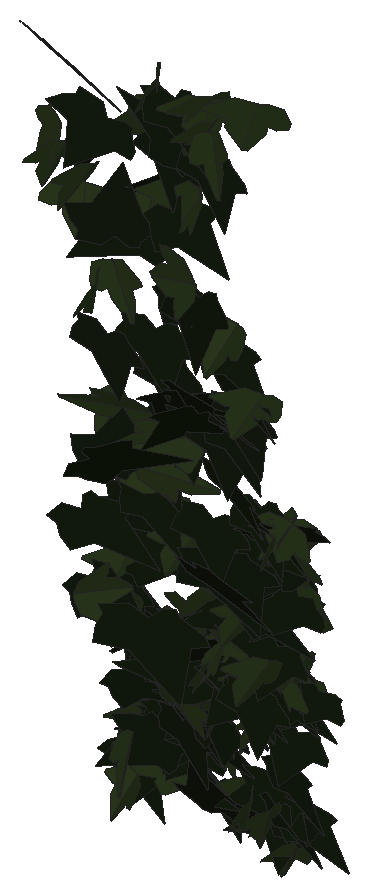
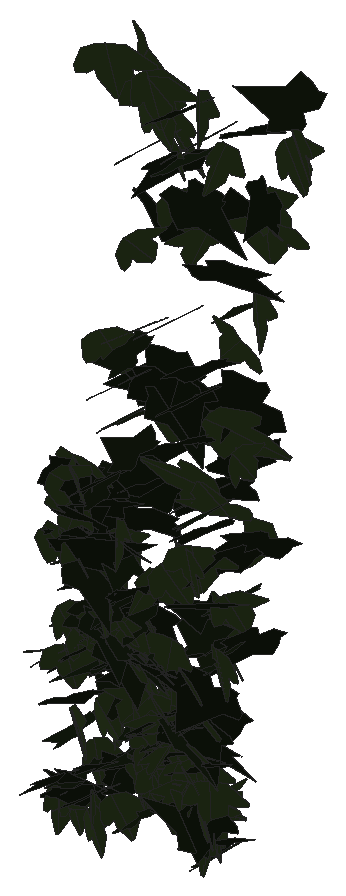
# SketchUp Ruby script. Lengths in millimetres.
U = 1.mm
M = Sketchup.active_model
def pt(a) = Geom::Point3d.new(a.map { |v| v * U })
def face(e, loops, mat)
  f = e.add_face(loops[0].map { |a| pt(a) })
  loops[1..].each { |l| e.add_face(l.map { |a| pt(a) }).erase! }
  f.material = f.back_material = mat if mat
  f
end
# faces: each face lists its corners as indices into pts; further lists are holes
def faces(e, pts, list, mat = nil) = list.each { |f| face(e, (f[0].is_a?(Array) ? f : [f]).map { |l| l.map { |i| pts[i] } }, mat) }
# xy, xz, yz: faces in a plane at the given z, y or x. An outline is a flat list of corners, or four numbers for a rectangle; further outlines are holes
def ring(l) = l.size == 4 ? [[l[0], l[1]], [l[2], l[1]], [l[2], l[3]], [l[0], l[3]]] : l.each_slice(2).to_a
def flat(e, list, mat, &to3) = list.each { |f| face(e, (f[0].is_a?(Array) ? f : [f]).map { |l| ring(l).map { |u, v| to3.(u, v) } }, mat) }
def xy(e, z, list, mat = nil) = flat(e, list, mat) { |x, y| [x, y, z] }
def xz(e, y, list, mat = nil) = flat(e, list, mat) { |x, z| [x, y, z] }
def yz(e, x, list, mat = nil) = flat(e, list, mat) { |y, z| [x, y, z] }
def lines(e, pts, list) = list.each { |a, b| e.add_line(pt(pts[a]), pt(pts[b])) }
# prism: a flat outline (further loops are holes) pulled along v
def prism(e, loops, v, mat = nil)
  f = face(e, loops, mat); d = Geom::Vector3d.new(v.map { |x| x * U })
  f.pushpull(f.normal.samedirection?(d) ? d.length : -d.length)
end
def box(e, o, s, mat = nil) = prism(e, [[o, [o[0] + s[0], o[1], o[2]], [o[0] + s[0], o[1] + s[1], o[2]], [o[0], o[1] + s[1], o[2]]]], [0, 0, s[2]], mat)
def at(x, y, z, deg = 0) = Geom::Transformation.translation(pt([x, y, z])) * Geom::Transformation.rotation(ORIGIN, Z_AXIS, deg.degrees)
def axes(o, x, y, z) = Geom::Transformation.new([*x, 0, *y, 0, *z, 0, *pt(o).to_a, 1])
def part(name) = M.definitions.add(name)
# library, detail: a bought-in or finely detailed component or shape, given as its bounding box
def library(name, o, s) = part(name).tap { |d| box(d.entities, o, s) }
def detail(e, o, s) = box(e.add_group.entities, o, s)
def put(e, d, t, mat = nil) = e.add_instance(d, t).tap { |i| i.material = mat if mat }
def group(e, t, mat = nil) = e.add_group.tap { |g| g.transformation = t; g.material = mat if mat }.entities
root = M.entities
M.materials.add("efeu1").color = [18, 25, 13]
M.materials.add("efeu2").color = [43, 57, 29]
c1 = part("ivyleaf_10")
p = [[0,12.8,-0.8],[-1.5,51.3,-10.9],[-4.9,51,-11.6],[-13.6,26.5,-7.3],[-13.2,15.9,-4.6],[-21.1,19.3,-7.2],
  [-29.5,16.3,-8.3],[-29.2,8.3,-6.2],[-19.7,-9.8,0.5],[-7.6,-13,4],[1,-12.2,5.8],[-0.4,51.1,-11.1],
  [-1.5,51.1,-10.9],[1,-12.4,5.9],[16.9,-12.4,3.5],[35.1,9.1,-5.1],[35,12.9,-6.1],[20.5,16.4,-4.9],
  [15.8,15,-3.8],[15.3,27.6,-7.1],[12.8,31.3,-7.8]]
faces(c1.entities,p,[[0,1,2,3,4,5,6,7,8,9,10],[11,12,0,13,14,15,16,17,18,19,20]],"efeu2")
c2 = part("ivyleaf_9")
p = [[39.1,54.8,31.7],[34.5,51.8,30.2],[-5.3,25.2,17.3],[-17.9,28.3,20.9],[-21.6,21.7,17],[-20.2,4.3,5.3],
  [-22.9,-0.3,2.5],[-17.1,-4,-0.6],[-2,-2.1,-1.2],[-0.7,-15.4,-10.1],[16.6,-22.3,-16.7],[21.1,-15.1,-12.5],
  [32.7,-10.7,-11],[46.1,-1.8,-6.6],[30.8,11.2,3.8]]
faces(c2.entities,p,[[0,1,2,3,4,5,6,7,8,9,10,11,12,13,14]],"efeu1")
put(root,c1,axes([1434.4,970.3,1660.3],[-1.04964,0.5725,0.28622],[-0.43851,0.17492,-0.79383],[-1.1365,-0.59623,0.04194]))
put(root,c2,axes([1417.1,894.4,1905.8],[0.23864,-0.56618,-0.78224],[-0.27175,0.76926,-0.57968],[1.8176,0.18935,0.01604]))
put(root,c2,axes([1415.3,969.2,1644.3],[0.27967,-0.82614,-0.05758],[-0.01819,0.05678,-0.83911],[1.57602,0.14726,0.00053]))
put(root,c1,axes([1435.7,960,1718.2],[-1.01449,-0.6751,-0.06263],[0.06682,0.05208,-0.86016],[1.28864,-0.53418,-0.0047]))
put(root,c1,axes([1431.5,964.2,1672.8],[0.35686,-0.82142,0.0966],[0.12958,-0.08338,-0.84121],[1.56876,0.19375,0.04751]))
put(root,c2,axes([1429.2,970.8,1655.9],[-0.76095,-0.73239,0.12628],[0.0387,-0.15413,-0.82948],[1.41392,-0.38994,0.09067]))
put(root,c2,axes([1396.9,838,2598.5],[0.91673,-0.76677,0.5409],[0.7383,-0.3909,-0.89958],[1.62613,0.60974,0.1035]))
put(root,c1,axes([1433.1,943.4,1890.3],[1.07356,-0.65991,-0.22821],[0.00287,0.29452,-0.84794],[1.32891,0.53247,0.18619]))
put(root,c2,axes([1442.1,845.9,2471],[-0.26448,0.20363,-0.96166],[-1.08746,0.77356,0.24637],[1.5223,0.58798,0.00891]))
put(root,c1,axes([1441.2,790,2530.7],[0.91565,-0.84518,-0.38706],[-0.21709,0.37886,-0.96906],[1.75584,0.4876,0.08203]))
put(root,c1,axes([1438,968.2,1685.2],[0.3553,-0.82918,0.02072],[0.01414,-0.01956,-0.84994],[1.57853,0.18681,0.00295]))
put(root,c1,axes([1444.9,957.2,1685.3],[-0.56888,-0.76943,0.24282],[-0.09597,-0.24063,-0.82455],[1.53256,-0.30068,0.0385]))
put(root,c1,axes([1445.2,840.3,2455],[-0.07469,-0.99115,0.30908],[-0.05688,-0.30809,-0.99178],[1.97513,-0.04635,-0.01687]))
put(root,c1,axes([1446.4,793.8,2506.2],[-0.23783,-1.02613,0.13782],[0.04918,-0.14187,-1.03284],[1.96986,-0.12035,0.04243]))
put(root,c1,axes([1439.1,900.2,2138.7],[-0.19002,-0.7118,0.60771],[0.39442,-0.6128,-0.68372],[1.73705,0.06128,0.22173]))
put(root,c2,axes([1447.4,964.6,1693.6],[0.96749,0.62386,-0.24385],[-0.49824,-0.09672,-0.79322],[-1.17341,0.55545,0.13575]))
put(root,c1,axes([1451.5,901.3,1940.8],[-0.72211,-0.75499,0.40283],[0.11994,-0.46411,-0.81048],[1.62421,-0.30139,0.23894]))
put(root,c1,axes([1441.6,842.8,2424],[1.7773,0.33849,0.00534],[0.00811,0.00391,-0.9933],[-0.64424,0.93386,0.00222]))
put(root,c2,axes([1436.8,899.8,2012.8],[0.5542,-0.31754,-0.82236],[-0.35804,0.82372,-0.38468],[1.63909,0.2873,0.19402]))
put(root,c2,axes([1443.1,948.5,1850.1],[1.40022,0.45952,-0.05842],[-0.09682,-0.02883,-0.86743],[-0.87627,0.73747,0.00249]))
put(root,c1,axes([1487.6,870.2,2154.6],[0.4405,0.36401,-0.91335],[-1.86951,0.12612,-0.19866],[0.08078,0.93374,0.3829]))
put(root,c1,axes([1458.6,839.2,2313.9],[0.18528,-0.93087,-0.39747],[0.05517,0.40171,-0.93369],[1.92559,0.07806,0.065]))
put(root,c1,axes([1460,954,1736.2],[-0.91075,-0.72045,-0.03433],[0.07,0.01677,-0.86464],[1.37094,-0.47947,0.02135]))
put(root,c2,axes([1433.3,857.4,2014.5],[0.29722,-0.55902,-0.7958],[0.35513,0.80824,-0.53115],[1.81652,-0.06654,0.23405]))
put(root,c2,axes([1441.5,973.3,1666.6],[0.20326,0.8293,-0.08372],[0.05259,0.08083,0.83598],[1.58548,-0.109,-0.01699]))
put(root,c1,axes([1436.5,902.7,2297.3],[1.35088,-0.33728,0.56936],[1.03127,-0.18308,-0.78396],[0.72299,0.89132,0.05442]))
put(root,c2,axes([1441.7,930.8,1886.7],[0.26193,-0.86894,0.15465],[0.05449,-0.15204,-0.87976],[1.67887,0.1405,0.00443]))
put(root,c2,axes([1446.7,949.7,1809.2],[0.32729,-0.86263,-0.07627],[-0.03067,0.07456,-0.87961],[1.64789,0.17272,-0.00122]))
put(root,c2,axes([1486.9,892,2377.5],[-1.65754,-0.3691,0.27433],[-0.49297,-0.09177,-0.94578],[0.72323,-0.90849,-0.01592]))
put(root,c2,axes([1478.5,939.4,1782.8],[0.29328,0.79954,-0.30007],[-0.29361,-0.27384,-0.80887],[-1.59859,0.19698,0.09351]))
put(root,c1,axes([1472.3,957.7,1698.3],[-0.92655,-0.69222,0.04256],[-0.03708,-0.03833,-0.84625],[1.3194,-0.48719,0.0061]))
put(root,c1,axes([1496,935,1675.2],[0.19709,0.03091,-0.87008],[-1.64931,-0.08056,-0.106],[-0.15927,0.87251,0.02104]))
put(root,c2,axes([1466.5,965.1,1737],[-0.73514,-0.74123,0.18677],[-0.17365,-0.16306,-0.83582],[1.4444,-0.39686,-0.00543]))
put(root,c2,axes([1488.2,960.4,1782.7],[-0.83597,0.74291,-0.00144],[0.00586,0.00015,-0.86304],[-1.4139,-0.43925,-0.00273]))
put(root,c1,axes([1472.1,963.3,1733],[-0.87648,-0.7133,-0.13305],[0.18693,0.09486,-0.84849],[1.36825,-0.46989,0.03069]))
put(root,c1,axes([1465.8,894.8,1666.3],[-0.2456,-0.44674,0.81263],[0.51462,-0.80293,-0.39847],[1.6882,0.17977,0.23969]))
put(root,c2,axes([1474.5,940.5,1948.6],[-1.1317,-0.64309,0.21061],[0.00802,-0.28389,-0.85492],[1.28787,-0.56334,0.1904]))
put(root,c2,axes([1457,912.2,1796.5],[0.15487,-0.18572,-0.95521],[-0.06411,0.95743,-0.18902],[1.85089,0.0487,0.07338]))
put(root,c1,axes([1480.8,935.1,2009.9],[-1.28263,-0.59584,0.15556],[0.02437,-0.24412,-0.87957],[1.17175,-0.64714,0.18857]))
put(root,c1,axes([1471.4,965.9,1714.4],[0.50447,0.78867,0.19855],[0.01441,0.20643,-0.83007],[-1.54777,0.25898,0.05699]))
put(root,c2,axes([1482.8,829.5,2538.4],[-1.0304,-0.75563,0.39473],[-0.24607,-0.38942,-0.92279],[1.60375,-0.54524,0.11202]))
put(root,c2,axes([1477,844.4,2095.4],[-0.86528,-0.37518,0.81195],[1.29354,0.44717,0.5872],[-1.10659,0.81608,0.05152]))
put(root,c2,axes([1462.6,929.5,2072],[0.40961,-0.88862,-0.13844],[-0.01827,0.14007,-0.91402],[1.71153,0.21417,0.02338]))
put(root,c1,axes([1481.6,949,1850.4],[0.9459,-0.73368,0.01446],[0.02477,-0.00865,-0.88615],[1.39639,0.49714,0.00592]))
put(root,c2,axes([1465.3,878.6,1929.5],[0.09638,-0.90044,0.13314],[0.08654,-0.13068,-0.90108],[1.7302,0.0567,0.03766]))
put(root,c1,axes([1467.9,894.7,2057.6],[1.66542,0.12632,-0.31002],[0.5173,0.23843,0.86434],[0.37194,-0.89722,0.18604]))
put(root,c1,axes([1481.6,876,2525.4],[-0.29444,-0.76586,-0.63412],[0.42807,0.59816,-0.7773],[1.84331,-0.26124,0.07922]))
put(root,c2,axes([1470.1,944.1,1854.7],[-0.03623,-0.8479,0.2664],[0.14076,-0.26705,-0.84468],[1.68563,0.00408,0.07626]))
put(root,c1,axes([1490.8,954.4,1688.4],[-1.35071,-0.4691,-0.00957],[0.01554,0.005,-0.85073],[0.89284,-0.70975,0.00033]))
put(root,c1,axes([1473.2,960.6,1731.9],[0.97081,-0.51401,0.45366],[0.64493,-0.30252,-0.72379],[1.13426,0.61195,0.02325]))
put(root,c2,axes([1498.2,954.2,1743.3],[-1.38987,-0.41323,0.17129],[-0.16559,-0.19045,-0.8304],[0.83508,-0.72552,0.12042]))
put(root,c2,axes([1510.6,894.3,1736.5],[-1.64683,0.01971,0.04934],[-0.09342,0.01165,-0.86545],[-0.03871,-0.86662,-0.01051]))
put(root,c2,axes([1472.1,946.1,1800.7],[0.41559,-0.83992,-0.13754],[0.05075,0.14867,-0.86559],[1.61902,0.21094,0.06244]))
put(root,c1,axes([1465.2,884.4,1899.4],[0.82946,-0.26126,0.83715],[1.45325,-0.34669,-0.50572],[0.82083,0.87782,0.04942]))
put(root,c1,axes([1498.4,930.9,2004.9],[1.07405,-0.68067,-0.24253],[-0.16028,0.24368,-0.87985],[1.36586,0.56385,0.08747]))
put(root,c1,axes([1491.8,956.9,1760.9],[1.62328,-0.14206,-0.02323],[-0.04513,-0.00095,-0.86466],[0.27022,0.85324,-0.00483]))
put(root,c2,axes([1479.1,919.9,2083.7],[0.2075,-0.92058,-0.06337],[0.01437,0.0647,-0.92689],[1.75614,0.10824,0.01507]))
put(root,c1,axes([1498.3,936.6,1785.3],[-1.52837,-0.32335,-0.1119],[0.19436,0.04596,-0.8657],[0.62153,-0.80951,-0.00446]))
put(root,c2,axes([1498.1,828.2,2401.8],[-1.21499,-0.40319,0.70228],[1.20254,0.3113,0.7531],[-0.96392,0.89657,0.05433]))
put(root,c1,axes([1494,788.4,1960.7],[0.06546,0.13379,1.09212],[-0.13984,1.09049,-0.13128],[-2.08938,-0.06879,0.043]))
put(root,c2,axes([1483.4,907.7,2035],[0.11537,-0.8883,-0.25008],[0.03162,0.25162,-0.88977],[1.75604,0.05383,0.03245]))
put(root,c2,axes([1501.5,956,1724.2],[-0.92501,-0.68308,0.11872],[-0.09382,-0.11057,-0.83801],[1.31619,-0.48795,0.0237]))
put(root,c1,axes([1507.5,966.8,1716.4],[-0.95439,-0.66753,0.15686],[-0.05818,-0.17238,-0.83128],[1.30375,-0.49635,0.07774]))
put(root,c2,axes([1480.7,899.8,1882.1],[0.40991,-0.81471,0.45489],[0.41271,-0.41037,-0.83764],[1.72725,0.2914,0.09219]))
put(root,c2,axes([1525.6,884.9,2458.9],[-0.53775,0.7891,-0.54165],[-0.00776,-0.56575,-0.82208],[-1.82156,-0.23055,0.16341]))
put(root,c2,axes([1507,962.7,1702.3],[-0.93225,-0.60352,0.33809],[-0.02156,-0.40721,-0.74332],[1.31639,-0.43407,0.22725]))
put(root,c1,axes([1513,943.9,1879.4],[-1.4834,0.38853,0.11578],[-0.23402,0.01252,-0.86982],[-0.73524,-0.78787,0.04327]))
put(root,c1,axes([1502.4,964.6,1752.3],[0.08807,0.85295,0.0692],[0.01301,0.06893,-0.8542],[-1.62862,0.04668,-0.00308]))
put(root,c1,axes([1515.7,938.5,1974.7],[-0.69758,-0.77477,0.4371],[-0.02028,-0.46889,-0.84006],[1.6929,-0.32487,0.17005]))
put(root,c1,axes([1501.3,890,2416.1],[0.6171,0.92853,0.11872],[0.02467,0.12118,-0.98313],[-1.7814,0.32333,0.02751]))
put(root,c2,axes([1498.7,901,2244.4],[-0.32905,-0.9389,-0.10082],[0.05503,0.09719,-0.95463],[1.79635,-0.17496,0.01078]))
put(root,c2,axes([1492.9,853.7,1870.9],[0.24376,0.95405,-0.29052],[-0.02416,0.29444,0.96133],[1.8979,-0.11879,0.04955]))
put(root,c2,axes([1508.7,947.7,1792.8],[-0.38927,-0.85126,0.02522],[-0.03907,-0.021,-0.87536],[1.62035,-0.20501,-0.01505]))
put(root,c2,axes([1502.7,960.2,1776.1],[-0.32992,-0.84195,-0.0494],[0.36895,0.0093,-0.83887],[1.56219,-0.18001,0.18769]))
put(root,c2,axes([1502.8,809.3,2280.3],[-0.14087,-0.94076,0.22442],[0.10811,-0.22892,-0.94088],[1.83753,-0.05865,0.07256]))
put(root,c1,axes([1520,869.5,2580.7],[0.15772,-0.88455,-0.49433],[0.12164,0.49955,-0.88318],[1.92468,0.04091,0.09633]))
put(root,c1,axes([1510.1,957,1785.8],[0.89566,0.7276,0.02766],[0.04432,0.01788,-0.86647],[-1.38505,0.47108,-0.00984]))
put(root,c2,axes([1507.7,911,2200.4],[-0.05042,-0.94817,0.06026],[-0.05488,-0.05946,-0.94815],[1.80736,-0.02826,-0.02711]))
put(root,c2,axes([1539.9,936.1,1853.5],[-1.31199,0.51075,-0.19193],[0.19098,-0.1853,-0.85353],[-1.02071,-0.69117,0.087]))
put(root,c1,axes([1551.2,870,2140.1],[0.9072,0.19364,-0.82272],[-1.51761,-0.21014,-0.51146],[-0.53333,0.92733,0.0559]))
put(root,c1,axes([1522.1,911.7,1783.9],[-1.40217,0.41996,-0.20628],[0.36595,-0.07902,-0.84764],[-0.8118,-0.76099,-0.02582]))
put(root,c2,axes([1516.8,957.9,1782.6],[-0.10107,-0.86174,-0.09082],[-0.01354,0.09142,-0.86328],[1.64908,-0.05206,-0.01265]))
put(root,c2,axes([1506.8,780.4,2139.5],[0.23389,0.59882,-0.92124],[0.20572,0.9159,0.60977],[2.08102,-0.15785,0.04326]))
put(root,c1,axes([1523.3,957.5,1813.6],[0.88738,-0.59261,0.43719],[0.47881,-0.35815,-0.75376],[1.31724,0.5294,-0.02054]))
put(root,c2,axes([1521.3,917.2,2139],[-0.31425,-0.92005,-0.12111],[0.03514,0.11973,-0.93474],[1.76579,-0.16612,-0.00295]))
put(root,c2,axes([1549.5,880.5,2504.4],[-0.44035,-0.96646,0.15669],[0.0664,0.15277,0.99377],[-1.86221,0.23398,-0.00162]))
put(root,c1,axes([1537.2,946.6,1760.8],[-0.73363,-0.74939,0.19121],[0.06349,-0.22955,-0.83242],[1.47056,-0.36394,0.13133]))
put(root,c1,axes([1538.3,949.8,1728.8],[-0.29447,-0.8501,0.0923],[0.01137,-0.09487,-0.86376],[1.62738,-0.15316,0.02274]))
put(root,c2,axes([1547.3,880.8,2170.9],[0.08015,0.93106,-0.20242],[-0.09256,-0.20026,-0.93122],[-1.81103,0.05144,0.03863]))
put(root,c1,axes([1541.7,887.6,2445.3],[-0.75847,-0.83351,0.36406],[-0.00462,-0.3965,-0.91043],[1.73105,-0.36627,0.15709]))
put(root,c2,axes([1517.1,945.1,1758.5],[0.3915,-0.83275,0.17944],[0.10617,-0.17104,-0.85769],[1.6178,0.21275,0.01286]))
put(root,c2,axes([1564.8,897.2,1830.9],[-1.08381,0.06456,0.67096],[-1.1579,-0.42736,-0.47525],[0.55227,-0.76931,0.32031]))
put(root,c1,axes([1502.7,891.2,2076.2],[0.11866,-0.00685,-0.9447],[1.74812,-0.22102,0.06222],[-0.42059,-0.9206,-0.00791]))
put(root,c2,axes([1533.5,952.3,1766.3],[-0.30897,-0.77343,0.35448],[-0.16711,-0.34372,-0.79016],[1.61059,-0.18403,-0.01399]))
put(root,c2,axes([1562.7,955.8,1843.5],[-1.61484,-0.07755,0.17646],[-0.32258,-0.07912,-0.84976],[0.17468,-0.86302,0.06205]))
put(root,c1,axes([1546.3,958.3,1712.3],[1.12512,-0.52975,-0.34968],[-0.15826,0.40909,-0.76035],[1.19765,0.55173,0.22802]))
put(root,c1,axes([1538.4,938.5,1783.7],[-0.31393,-0.8864,0.06493],[0.10039,0.05616,0.90066],[-1.68853,0.16814,0.04148]))
put(root,c1,axes([1549.6,943.8,1791.1],[-0.08842,-0.86798,-0.1242],[0.04488,0.12309,-0.86906],[1.66816,-0.04932,0.0168]))
put(root,c2,axes([1530.8,971.9,1653.7],[0.15553,-0.80698,0.22827],[0.114,-0.22315,-0.81032],[1.59204,0.09481,0.03572]))
put(root,c2,axes([1560.3,878.2,2193.7],[0.52567,0.79679,-0.45461],[-0.40902,-0.40536,-0.84104],[-1.69734,0.34445,0.06188]))
put(root,c1,axes([1533.5,957.5,1809.3],[1.0795,0.5549,0.35523],[0.38908,0.29737,-0.79095],[-1.19206,0.59956,0.06353]))
put(root,c2,axes([1532,905.1,2298.8],[0.44561,-0.89814,-0.26951],[-0.00887,0.27666,-0.92603],[1.78461,0.22563,0.06269]))
put(root,c2,axes([1534.3,904.5,1761],[0.26022,-0.89736,0.27387],[0.06686,-0.27167,-0.9077],[1.78437,0.14104,-0.00593]))
put(root,c2,axes([1541.6,880.9,2493.7],[-0.34356,-0.88959,0.42906],[0.02314,-0.43814,-0.90329],[1.87956,-0.15721,0.08955]))
put(root,c1,axes([1563.3,975.4,1662.8],[-0.56658,-0.75396,0.19789],[-0.09356,-0.19325,-0.81024],[1.48059,-0.30073,0.02453]))
put(root,c2,axes([1537.6,942.2,1733.5],[1.08491,-0.55363,-0.32653],[-0.16169,0.36772,-0.77178],[1.21255,0.54438,0.18924]))
put(root,c2,axes([1558.8,951.9,1840.4],[-1.13871,-0.64533,0.00139],[0.18758,-0.09325,-0.8695],[1.21379,-0.591,0.13567]))
put(root,c2,axes([1569.5,950.9,1858.1],[0.21076,0.8712,0.03362],[-0.09416,0.04011,-0.87654],[-1.65662,0.10856,0.0541]))
put(root,c1,axes([1561.6,923.8,1780.8],[0.48183,-0.7476,-0.35306],[0.0676,0.37874,-0.77649],[1.57206,0.21285,0.1416]))
put(root,c2,axes([1584.6,948.7,1871.5],[-0.88253,0.74719,-0.10557],[-0.058,-0.14235,-0.87365],[-1.43501,-0.45377,0.10024]))
put(root,c2,axes([1546.8,874.6,2562.9],[0.11178,-0.99008,-0.17126],[0.05615,0.17318,-0.99104],[1.91147,0.05281,0.03913]))
put(root,c1,axes([1552.7,780.1,1796.7],[0.9358,-0.77823,0.62119],[0.71001,-0.49837,-0.91964],[1.75708,0.61586,0.04077]))
put(root,c1,axes([1560.5,907.7,1936.5],[-0.36745,-0.61993,-0.68087],[0.52032,0.62571,-0.64723],[1.67346,-0.33067,0.05174]))
put(root,c2,axes([1553,945.5,1753.3],[-0.21531,-0.71017,0.49254],[0.14471,-0.50299,-0.70778],[1.63847,-0.0489,0.12723]))
put(root,c1,axes([1566.9,900.7,1844.4],[0.34101,-0.85594,0.12987],[0.16229,-0.11453,-0.87248],[1.63966,0.18935,0.05934]))
put(root,c2,axes([1572.3,923,1657.3],[1.28241,-0.38153,0.53566],[-0.85497,0.29309,0.77384],[-0.91413,-0.80936,0.02771]))
put(root,c2,axes([1582.6,902.7,1879.9],[-0.19688,0.71078,-0.53068],[-0.04576,-0.53633,-0.71366],[-1.68759,-0.06838,0.08126]))
put(root,c2,axes([1560.7,953.4,1833.8],[-0.48901,-0.83225,-0.11632],[0.02589,0.1175,-0.87074],[1.59912,-0.2564,-0.02147]))
put(root,c2,axes([1586.3,862,2187.4],[-0.0393,0.64551,-0.73056],[-0.1214,-0.73006,-0.64326],[-1.85143,0.03417,0.05769]))
put(root,c1,axes([1569.9,954.2,1849.6],[1.29593,-0.5423,-0.10008],[0.01607,0.16925,-0.85968],[1.04941,0.6671,0.13676]))
put(root,c2,axes([1554.4,938.8,1895.5],[1.04726,-0.69072,-0.10987],[-0.01971,0.13173,-0.88005],[1.33095,0.54544,0.07342]))
put(root,c1,axes([1582.6,948.8,1865.4],[-0.53862,-0.82945,0.11986],[0.02581,-0.13103,-0.87469],[1.59479,-0.27801,0.05464]))
put(root,c2,axes([1596.1,939,1911.1],[-0.86303,-0.42712,0.63768],[-0.90672,-0.42406,-0.62282],[1.14525,-0.65761,-0.01256]))
put(root,c2,axes([1549.1,871.5,2199.1],[1.65568,-0.31244,0.24362],[0.43933,-0.07799,-0.92434],[0.61282,0.90004,0.00448]))
put(root,c2,axes([1570.5,951.9,1849.1],[-0.19868,-0.87209,-0.07403],[-0.00169,0.07466,-0.87827],[1.66574,-0.10394,-0.00972]))
put(root,c2,axes([1573.2,922.4,1686.2],[1.40386,-0.27403,-0.46755],[-0.79397,0.21694,-0.7853],[0.65836,0.84596,0.04993]))
put(root,c1,axes([1584.6,895.6,1874.4],[0.87977,-0.76046,0.01149],[0.01143,-0.0098,-0.88993],[1.44743,0.4623,0.00004]))
put(root,c2,axes([1598,946.6,1878.4],[0.11215,0.86877,0.1688],[-0.04388,0.17062,-0.87011],[-1.6838,0.05342,0.03392]))
put(root,c1,axes([1594,868.8,2548.8],[-0.23292,-0.98728,0.13819],[-0.06268,-0.13515,-0.99471],[1.89628,-0.12573,-0.0159]))
put(root,c1,axes([1594.8,872.2,2581.1],[-0.61895,-0.96677,0.02313],[-0.01439,-0.02186,-1.02],[1.84042,-0.3253,-0.00019]))
put(root,c1,axes([1579.9,951.3,1888.6],[-1.54687,-0.06604,-0.34802],[0.66097,0.02289,-0.81543],[0.1327,-0.88385,0.00488]))
put(root,c1,axes([1595.3,872,2574.1],[-1.26054,-0.76235,0.1255],[0.10163,-0.21008,-0.9943],[1.46692,-0.64054,0.17673]))
put(root,c1,axes([1592.1,944.5,1887.7],[1.22442,-0.61121,-0.06337],[-0.07439,0.05086,-0.88734],[1.16712,0.64446,0.00993]))
put(root,c1,axes([1585.3,944.1,1868],[0.20647,0.81259,0.30422],[0.00997,0.30597,-0.81913],[-1.65131,0.10345,0.03309]))
put(root,c1,axes([1594.7,932.2,2003.2],[0.2126,-0.75215,-0.48219],[0.08035,0.48985,-0.75431],[1.69849,0.07097,0.09604]))
put(root,c1,axes([1598.5,947.8,1887.3],[0.17182,-0.88256,-0.05683],[-0.00015,0.05711,-0.88715],[1.68317,0.0901,0.00572]))
put(root,c1,axes([1599.5,976.9,1630.6],[0.0361,-0.82787,-0.03557],[0.00191,0.0356,-0.82808],[1.57705,0.01891,0.00182]))
put(root,c1,axes([1599.6,955.9,1770.6],[0.1379,-0.88468,0.28141],[0.08109,-0.2788,-0.88744],[1.76499,0.08193,0.01878]))
put(root,c1,axes([1630.2,933.9,1858.9],[-0.25789,0.04894,0.8868],[-1.69005,-0.02342,-0.1344],[0.03006,-0.89678,0.0519]))
put(root,c1,axes([1611.8,924.8,1869.3],[-1.09845,-0.60238,0.2892],[-0.17004,-0.30914,-0.82223],[1.2603,-0.56673,0.14112]))
put(root,c2,axes([1592.5,883.1,2045.6],[-0.30631,-0.9143,0.00882],[-0.00255,-0.00872,-0.92836],[1.74017,-0.16095,0.00019]))
put(root,c2,axes([1582.7,945.7,1776.2],[0.07749,-0.56712,0.6413],[0.44506,-0.61024,-0.5545],[1.56736,0.20132,0.12575]))
put(root,c1,axes([1605.6,946.5,1894.8],[-0.9711,0.72885,0.03261],[-0.15353,-0.01682,-0.88648],[-1.38001,-0.51101,0.07568]))
put(root,c2,axes([1590.1,822,2460.7],[0.30411,-0.74998,-0.71436],[-0.22844,0.70453,-0.76651],[1.95795,0.19869,0.02152]))
put(root,c2,axes([1582.1,895,1834.5],[1.3338,-0.53811,0.023],[0.04739,-0.00533,-0.88351],[1.02396,0.70118,0.01093]))
put(root,c1,axes([1607.1,965.1,1651.4],[0.38751,-0.72912,-0.36426],[0.12203,0.38862,-0.74203],[1.54638,0.15204,0.14984]))
put(root,c2,axes([1593.4,881.3,2499.5],[-0.04096,-0.98939,0.15928],[-0.05672,-0.15861,-0.98928],[1.90641,-0.02598,-0.02601]))
put(root,c2,axes([1596.1,900.4,2143.2],[-0.27335,-0.88816,0.27106],[0.04568,-0.27774,-0.89734],[1.76672,-0.13023,0.06514]))
put(root,c2,axes([1592.5,915.9,2151.9],[0.22994,-0.9372,-0.04866],[-0.00298,0.04886,-0.94495],[1.78609,0.12074,0.00469]))
put(root,c1,axes([1613.9,819.5,2484.8],[1.0296,-0.89201,-0.14499],[-0.13992,0.12498,-1.04324],[1.71425,0.54595,0.00193]))
put(root,c2,axes([1593.7,898.2,2260.5],[0.45459,-0.888,-0.27966],[0.1105,0.30236,-0.9105],[1.76843,0.20937,0.12878]))
put(root,c2,axes([1630.3,957.1,1679.4],[-1.05248,-0.29719,0.58866],[-0.70809,-0.49369,-0.59876],[1.0362,-0.63923,0.18875]))
put(root,c2,axes([1603.3,925.2,1837],[-0.42154,-0.76154,-0.47931],[0.28208,0.456,-0.79299],[1.68915,-0.2662,0.01281]))
put(root,c2,axes([1589.5,944.5,1906],[1.06132,-0.68675,0.12788],[0.3,-0.0357,-0.8791],[1.29519,0.57101,0.09883]))
put(root,c2,axes([1593.2,902,2091.8],[0.45039,-0.79116,0.44836],[0.33324,-0.41498,-0.82468],[1.69834,0.29124,0.04291]))
put(root,c2,axes([1627.2,910.6,1840],[-1.26228,-0.5663,0.16308],[-0.22858,-0.11048,-0.8721],[1.09805,-0.674,0.00593]))
put(root,c2,axes([1596.8,902.3,2226.4],[0.84137,-0.84127,0.09918],[0.06062,-0.09528,-0.95022],[1.61105,0.44294,-0.01604]))
put(root,c2,axes([1630.5,894,1951],[0.37295,0.77834,0.42438],[-0.1257,0.44623,-0.78792],[-1.68253,0.13919,0.15293]))
put(root,c2,axes([1648.8,943.8,1957.9],[-0.1525,-0.00309,0.89127],[-1.68884,-0.08346,-0.08007],[0.15873,-0.89097,0.00441]))
put(root,c2,axes([1601.9,942.8,1835.4],[1.15848,-0.52528,-0.38295],[-0.20772,0.43459,-0.76961],[1.21962,0.57297,0.23267]))
put(root,c2,axes([1637.4,942.7,1938.3],[-0.2395,0.88894,0.02665],[-0.00382,0.02663,-0.8978],[-1.69258,-0.12584,-0.00174]))
put(root,c2,axes([1609.4,749.9,1984],[-0.74371,-0.89375,-0.59578],[0.47395,0.54133,-0.97539],[1.98857,-0.46327,0.00965]))
put(root,c2,axes([1613.8,901.1,1842.3],[0.96724,-0.64767,-0.5035],[-0.5108,0.42842,-0.82201],[1.47539,0.57293,0.0455]))
put(root,c2,axes([1654.5,959.8,1661],[-1.57106,0.08718,0.2087],[-0.40101,-0.00937,-0.82951],[-0.15645,-0.8514,0.0305]))
put(root,c2,axes([1613.1,878.1,2001.8],[-0.85782,-0.54286,-0.6934],[0.9476,0.4854,-0.70366],[1.3824,-0.66959,0.05207]))
put(root,c2,axes([1615,905.6,2182.8],[0.02403,-0.94916,0.04458],[0.00928,-0.04452,-0.94923],[1.8084,0.01284,0.00428]))
put(root,c2,axes([1621.4,968.6,1648.2],[-0.3365,-0.86487,0.23013],[-0.06401,-0.22799,-0.88267],[1.7021,-0.17956,0.0123]))
put(root,c1,axes([1633.4,965.3,1749.5],[0.47534,-0.79859,-0.19078],[-0.05141,0.19131,-0.83617],[1.56179,0.24935,0.03054]))
put(root,c2,axes([1608.5,950.4,1895.7],[0.99007,-0.71243,-0.06599],[0.00706,0.08428,-0.88058],[1.36168,0.51757,0.05255]))
put(root,c1,axes([1640.7,883.4,1950.2],[-0.45301,-0.78157,0.42887],[-0.06447,-0.43564,-0.81272],[1.69549,-0.22539,0.08368]))
put(root,c2,axes([1631.3,971.9,1657.4],[-0.73977,-0.7385,-0.0891],[0.0613,0.08373,-0.83449],[1.41439,-0.38989,-0.01044]))
put(root,c2,axes([1665.9,934.9,1999.1],[-1.55159,0.2185,0.32741],[-0.61742,0.0535,-0.84349],[-0.42428,-0.87691,0.03012]))
put(root,c1,axes([1645.2,905.9,1856.2],[-1.04075,-0.69843,0.08079],[-0.10897,-0.05777,-0.88699],[1.33367,-0.54975,-0.00943]))
put(root,c1,axes([1639.6,946.9,1852.6],[-0.48081,-0.70248,0.58259],[0.15971,-0.61982,-0.71098],[1.72956,-0.13805,0.22761]))
put(root,c2,axes([1628.1,812.2,2368.4],[-1.26169,0.00185,-0.81514],[1.54111,-0.1192,-0.65882],[-0.17821,-1.0439,0.07378]))
put(root,c2,axes([1642.8,928.4,2018.8],[-1.08563,-0.69898,0.19822],[-0.15185,-0.19023,-0.90039],[1.37439,-0.57314,0.0571]))
put(root,c1,axes([1644.3,911.7,1680.9],[-0.32164,-0.85058,-0.14809],[0.04408,0.14637,-0.86719],[1.64258,-0.17048,-0.00573]))
put(root,c2,axes([1638.8,942.2,1981.3],[-0.88931,-0.7686,-0.07696],[0.04007,0.07724,-0.89922],[1.46956,-0.46722,-0.02205]))
put(root,c2,axes([1629.4,922.4,2054.6],[0.03809,-0.92729,-0.04151],[-0.0359,0.04111,-0.92733],[1.76622,0.02083,-0.01795]))
put(root,c2,axes([1620.9,926.2,2050.8],[0.96302,-0.7704,0.08751],[0.05308,-0.08634,-0.9214],[1.4747,0.5062,-0.02398]))
put(root,c2,axes([1628.1,943.9,1839.2],[0.42149,-0.7594,-0.41202],[-0.07123,0.41651,-0.78779],[1.64277,0.2129,0.07156]))
put(root,c1,axes([1653.8,883.6,2218.1],[-1.00084,-0.69764,0.39663],[-0.1184,-0.43734,-0.85172],[1.52274,-0.49254,0.19447]))
put(root,c2,axes([1621.5,826.1,2017.1],[1.91383,-0.22039,-0.07497],[-0.1387,0.01767,-1.02945],[0.42078,1.00822,0.00166]))
put(root,c1,axes([1668.3,735.2,2440.7],[0.67936,-0.56862,-0.94553],[-0.96776,0.79717,-0.67137],[1.86358,0.62126,-0.00395]))
put(root,c1,axes([1652.2,939.8,1962.3],[-0.43487,-0.87335,-0.01684],[0.02959,0.01334,-0.90267],[1.6622,-0.22872,0.01166]))
put(root,c1,axes([1653.3,958.5,1827.3],[-1.1108,-0.6183,0.17544],[0.03861,-0.25459,-0.82975],[1.22259,-0.55372,0.1856]))
put(root,c1,axes([1651.4,870.3,1715.5],[0.16673,-0.8972,-0.33867],[0.07509,0.34317,-0.8989],[1.8236,0.0679,0.06798]))
put(root,c2,axes([1630.3,954.1,1670.2],[0.69583,-0.76695,-0.06637],[-0.04931,0.06118,-0.84963],[1.46428,0.36652,0.00293]))
put(root,c1,axes([1654.5,944.8,1628.3],[-0.33151,-0.8244,-0.0312],[0.00798,0.031,-0.84259],[1.5701,-0.17422,-0.00231]))
put(root,c2,axes([1633,946.2,1851.9],[0.46664,-0.82456,-0.192],[-0.01954,0.19698,-0.85905],[1.61116,0.2412,0.04519]))
put(root,c2,axes([1661.4,911.9,2047.2],[0.79408,0.74755,-0.33083],[-0.35669,-0.27406,-0.85564],[-1.51439,0.45653,0.02806]))
put(root,c1,axes([1662.6,869.2,2593.8],[-1.4154,-0.67808,0.16239],[-0.04984,-0.21009,-0.99721],[1.32608,-0.73165,0.13585]))
put(root,c1,axes([1654.3,833.5,2326],[-0.51571,-0.67442,0.73419],[0.3501,-0.78158,-0.65007],[1.86478,-0.03977,0.32509]))
put(root,c1,axes([1657,905.7,2033.5],[0.39615,-0.84209,-0.33055],[0.14566,0.35436,-0.85456],[1.71554,0.16437,0.14889]))
put(root,c2,axes([1654.2,953.8,1767.4],[-0.71684,-0.75517,0.19103],[-0.04296,-0.20152,-0.84114],[1.48189,-0.37114,0.06803]))
put(root,c2,axes([1635.7,892.4,1953.5],[0.95759,-0.64277,-0.39943],[-0.01551,0.47503,-0.77469],[1.4402,0.43249,0.25724]))
put(root,c1,axes([1652.3,924.9,1840.4],[1.55711,-0.32092,0.07829],[0.13382,-0.03514,-0.87882],[0.61428,0.82114,-0.00701]))
put(root,c1,axes([1661.8,961.5,1633.5],[-0.36797,-0.77409,-0.25419],[0.11485,0.24693,-0.79787],[1.54639,-0.20254,-0.00123]))
put(root,c2,axes([1643,945.7,1724],[0.59946,-0.82423,-0.04069],[-0.016,0.04034,-0.88234],[1.5705,0.31502,0.00654]))
put(root,c1,axes([1665.7,925.4,2050.2],[0.56511,-0.87488,0.04478],[0.01501,-0.04461,-0.92387],[1.66718,0.29695,-0.00686]))
put(root,c1,axes([1667.1,928.4,2010.1],[-1.45471,0.4883,0.06405],[-0.09649,0.03961,-0.90699],[-0.93231,-0.766,-0.00607]))
put(root,c2,axes([1662.8,907.7,1899.3],[-0.7167,-0.77201,0.22239],[-0.04391,-0.23511,-0.85525],[1.52841,-0.36877,0.07971]))
put(root,c1,axes([1667.7,945.1,1869.2],[-0.21505,-0.81754,0.31871],[0.16729,-0.33027,-0.81603],[1.66159,-0.07256,0.12341]))
put(root,c1,axes([1681.2,931.3,2040.3],[-0.45058,-0.52738,0.70551],[-0.38998,-0.67753,-0.57523],[1.63042,-0.30781,0.05739]))
put(root,c1,axes([1649.8,806,2574.6],[1.21039,-0.53135,0.67206],[1.0326,-0.39797,-0.82808],[1.26191,0.83531,0.03298]))
put(root,c2,axes([1680.8,918.7,1965.2],[-1.265,-0.58662,0.14228],[-0.21282,-0.08831,-0.88648],[1.12894,-0.67397,-0.00769]))
put(root,c2,axes([1655.6,928.2,1835.9],[0.8391,-0.58927,-0.48643],[-0.28551,0.48391,-0.72219],[1.42593,0.44365,0.14164]))
put(root,c1,axes([1679,860.7,1901.3],[-0.51908,-0.85919,0.40955],[-0.03356,-0.4214,-0.89578],[1.81116,-0.25405,0.10078]))
put(root,c2,axes([1654.7,960.9,1664.5],[0.35733,-0.71682,-0.39271],[0.08591,0.41141,-0.72938],[1.55319,0.14216,0.13069]))
put(root,c1,axes([1702.1,927.7,1954.8],[-0.67557,0.16347,0.82727],[-1.53261,0.20065,-0.38518],[-0.47627,-0.87756,0.06603]))
put(root,c2,axes([1676.5,960.2,1826.1],[-1.0003,-0.59521,0.34471],[-0.04012,-0.41968,-0.75681],[1.30844,-0.4679,0.24032]))
put(root,c2,axes([1666.1,867.6,1855.7],[-0.33771,-0.86624,0.11328],[-0.00251,-0.11533,-0.88396],[1.66266,-0.17612,0.02167]))
put(root,c1,axes([1677.1,904.7,2053.6],[1.55533,-0.39496,-0.12894],[-0.20709,0.07113,-0.90751],[0.76314,0.82427,0.01653]))
